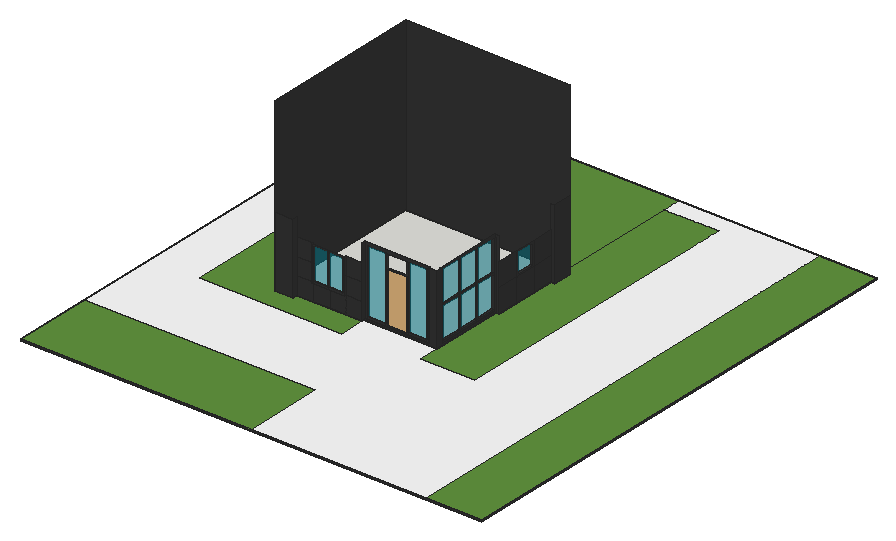
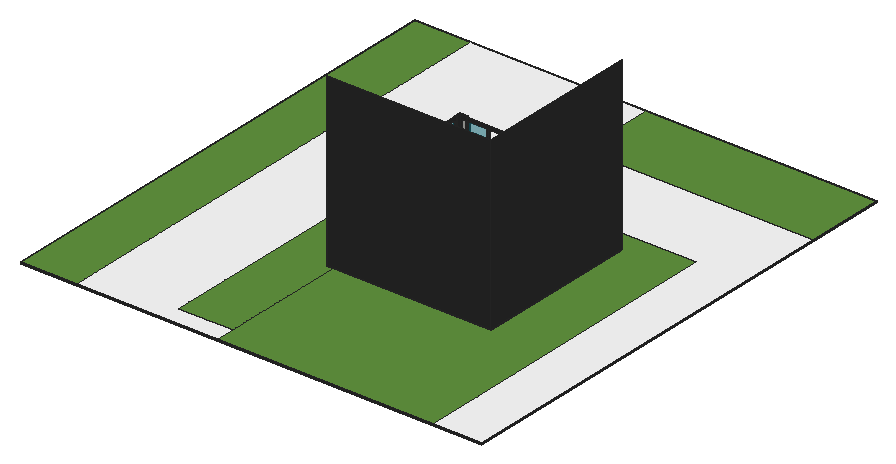
# SketchUp Ruby script. Lengths in inches.
U = 1.inch
M = Sketchup.active_model
def pt(a) = Geom::Point3d.new(a.map { |v| v * U })
def face(e, loops, mat)
  f = e.add_face(loops[0].map { |a| pt(a) })
  loops[1..].each { |l| e.add_face(l.map { |a| pt(a) }).erase! }
  f.material = f.back_material = mat if mat
  f
end
# faces: each face lists its corners as indices into pts; further lists are holes
def faces(e, pts, list, mat = nil) = list.each { |f| face(e, (f[0].is_a?(Array) ? f : [f]).map { |l| l.map { |i| pts[i] } }, mat) }
# xy, xz, yz: faces in a plane at the given z, y or x. An outline is a flat list of corners, or four numbers for a rectangle; further outlines are holes
def ring(l) = l.size == 4 ? [[l[0], l[1]], [l[2], l[1]], [l[2], l[3]], [l[0], l[3]]] : l.each_slice(2).to_a
def flat(e, list, mat, &to3) = list.each { |f| face(e, (f[0].is_a?(Array) ? f : [f]).map { |l| ring(l).map { |u, v| to3.(u, v) } }, mat) }
def xy(e, z, list, mat = nil) = flat(e, list, mat) { |x, y| [x, y, z] }
def xz(e, y, list, mat = nil) = flat(e, list, mat) { |x, z| [x, y, z] }
def yz(e, x, list, mat = nil) = flat(e, list, mat) { |y, z| [x, y, z] }
def lines(e, pts, list) = list.each { |a, b| e.add_line(pt(pts[a]), pt(pts[b])) }
# prism: a flat outline (further loops are holes) pulled along v
def prism(e, loops, v, mat = nil)
  f = face(e, loops, mat); d = Geom::Vector3d.new(v.map { |x| x * U })
  f.pushpull(f.normal.samedirection?(d) ? d.length : -d.length)
end
def box(e, o, s, mat = nil) = prism(e, [[o, [o[0] + s[0], o[1], o[2]], [o[0] + s[0], o[1] + s[1], o[2]], [o[0], o[1] + s[1], o[2]]]], [0, 0, s[2]], mat)
def at(x, y, z, deg = 0) = Geom::Transformation.translation(pt([x, y, z])) * Geom::Transformation.rotation(ORIGIN, Z_AXIS, deg.degrees)
def axes(o, x, y, z) = Geom::Transformation.new([*x, 0, *y, 0, *z, 0, *pt(o).to_a, 1])
def part(name) = M.definitions.add(name)
# library, detail: a bought-in or finely detailed component or shape, given as its bounding box
def library(name, o, s) = part(name).tap { |d| box(d.entities, o, s) }
def detail(e, o, s) = box(e.add_group.entities, o, s)
def put(e, d, t, mat = nil) = e.add_instance(d, t).tap { |i| i.material = mat if mat }
def group(e, t, mat = nil) = e.add_group.tap { |g| g.transformation = t; g.material = mat if mat }.entities
root = M.entities
M.materials.add("[0128_White]").color = [255, 255, 255]
M.materials.add("[0135_DarkGray]1").color = [53, 53, 53]
M.materials.add("[Grass Dark Green]").color = [97, 147, 63]
M.materials.add("[Translucent Glass Blue]1").color = [1, 149, 171]
M.materials["[Translucent Glass Blue]1"].alpha = 0.5
M.materials.add("[White Square Tile]").color = [255, 255, 255]
c1 = library("Glass door",[0,0,0],[43.79,7.72,89.79])
xy(root,-6,[[[0,0,1789.625,1912.5],[413.69,714.6875,485.69,714.6875,485.69,732.6875,738.69,732.6875,738.69,740.6875,1023.69,740.6875,1023.69,1026.6875,1035.69,1026.6875,1035.69,1278.6875,1049.69,1278.6875,1049.69,1350.6875,413.69,1350.6875]],[413.69,714.6875,413.69,1350.6875,1049.69,1350.6875,1049.69,1278.6875,1035.69,1278.6875,1035.69,1026.6875,1023.69,1026.6875,1023.69,740.6875,738.69,740.6875,738.69,732.6875,485.69,732.6875,485.69,714.6875]],"[0135_DarkGray]1")
xy(root,0,[[413.69,732.6875,738.69,732.6875,738.69,740.6875,1023.69,740.6875,1023.69,1350.6875,413.69,1350.6875]])
xy(root,0,[[413.69,714.6875,485.69,732.6875],[1023.69,1026.6875,1035.69,1026.6875,1035.69,1278.6875,1049.69,1278.6875,1049.69,1350.6875,1023.69,1350.6875]],"[0128_White]")
xy(root,0,[[0,0,894.8125,309.85],[1571.65,0,1789.625,1912.5],[[187.44,634.3125,738.69,634.3125,738.69,732.6875,485.69,732.6875,485.69,714.6875,413.69,714.6875,413.69,1350.6875,1023.69,1350.6875,1023.69,1912.5,187.44,1912.5],[413.69,714.6875,485.69,732.6875]],[1023.69,661.15,1235.57,661.15,1235.57,1840.4,1023.69,1840.4,1023.69,1350.6875,1049.69,1350.6875,1049.69,1278.6875,1035.69,1278.6875,1035.69,1026.6875,1023.69,1026.6875]],"[Grass Dark Green]")
xy(root,0,[[[894.8125,0,1571.65,0,1571.65,1912.5,1023.69,1912.5,1023.69,1840.4,1235.57,1840.4,1235.57,661.15,1023.69,661.15,1023.69,740.6875,738.69,740.6875,738.69,634.3125,187.44,634.3125,187.44,1912.5,0,1912.5,0,309.85,894.8125,309.85],[1023.69,1026.6875,1023.69,1350.6875,1049.69,1350.6875,1049.69,1278.6875,1035.69,1278.6875,1035.69,1026.6875]]],"[White Square Tile]")
xy(root,6,[[485.69,740.6875,738.69,745.6875]])
xy(root,6,[[738.69,740.6875,991.69,745.6875],[1018.69,762.6875,1023.69,1020.6875]],"[0135_DarkGray]1")
xy(root,12,[[750.69,745.6875,821.03,750.6875],[827.03,745.6875,903.36,750.6875],[909.36,745.6875,979.69,750.6875],[1013.69,774.6875,1018.69,856.6875],[1013.69,862.6875,1018.69,938.6875],
  [1013.69,944.6875,1018.69,1020.6875]],"[0135_DarkGray]1")
xy(root,67.89,[[548.94,728.6875,612.19,732.6875],[612.19,728.6875,675.44,732.6875]],"[0135_DarkGray]1")
xy(root,73.89,[[554.94,728.6875,609.19,732.6875],[615.19,728.6875,669.44,732.6875]],"[0135_DarkGray]1")
xy(root,96.52,[[1029.69,1116.6875,1035.69,1188.6875]],"[0135_DarkGray]1")
xy(root,132.78,[[1013.69,774.6875,1018.69,856.6875],[1013.69,862.6875,1018.69,938.6875],[1013.69,944.6875,1018.69,1020.6875]],"[0135_DarkGray]1")
xy(root,138.78,[[1013.69,774.6875,1018.69,856.6875],[1013.69,862.6875,1018.69,938.6875],[1013.69,944.6875,1018.69,1020.6875]],"[0135_DarkGray]1")
xy(root,175.04,[[1029.69,1116.6875,1035.69,1188.6875]],"[0135_DarkGray]1")
xz(root,0,[[0,-6,1789.625,0]],"[0135_DarkGray]1")
xz(root,714.6875,[[413.69,-6,485.69,0],[413.69,0,485.69,271.5625]],"[0135_DarkGray]1")
xz(root,728.6875,[[[548.94,67.89,675.44,203.67],[554.94,73.89,669.44,197.67]],[609.19,73.89,615.19,197.67]],"[0135_DarkGray]1")
xz(root,732.6875,[[485.69,-6,548.94,0],[548.94,-6,612.19,0],[612.19,-6,675.44,0],[675.44,-6,738.69,0],[485.69,0,548.94,67.89],
  [548.94,0,612.19,67.89],[612.19,0,675.44,67.89],[675.44,0,738.69,67.89],[485.69,67.89,548.94,135.78],[675.44,67.89,738.69,135.78],
  [485.69,135.78,548.94,203.67],[675.44,135.78,738.69,203.67]],"[0135_DarkGray]1")
xz(root,732.6875,[[554.94,73.89,609.19,197.67],[615.19,73.89,669.44,197.67]],"[Translucent Glass Blue]1")
xz(root,740.6875,[[738.69,-6,1023.69,0],[738.69,0,1023.69,0,1023.69,271.5625,991.69,271.5625,991.69,6,738.69,6]],"[0135_DarkGray]1")
xz(root,745.6875,[[[738.69,6,991.69,271.5625],[750.69,12,979.69,259.5625]],[821.03,12,827.03,12,827.03,204.96,903.36,204.96,903.36,12,909.36,12,909.36,259.5625,903.36,259.5625,903.36,211.2,827.03,211.2,827.03,259.5625,821.03,259.5625]],"[0135_DarkGray]1")
xz(root,750.6875,[[991.69,12,1001.69,259.5625]])
xz(root,750.6875,[[750.69,12,821.03,259.5625],[827.03,12,903.36,204.96],[909.36,12,979.69,259.5625]],"[Translucent Glass Blue]1")
xz(root,762.6875,[[1018.69,6,1023.69,271.5625]],"[0135_DarkGray]1")
xz(root,774.6875,[[1013.69,12,1018.69,132.78],[1013.69,138.78,1018.69,259.5625]],"[0135_DarkGray]1")
xz(root,856.6875,[[1013.69,12,1018.69,132.78],[1013.69,138.78,1018.69,259.5625]],"[0135_DarkGray]1")
xz(root,862.6875,[[1013.69,12,1018.69,132.78],[1013.69,138.78,1018.69,259.5625]],"[0135_DarkGray]1")
xz(root,938.6875,[[1013.69,12,1018.69,132.78],[1013.69,138.78,1018.69,259.5625]],"[0135_DarkGray]1")
xz(root,944.6875,[[1013.69,12,1018.69,132.78],[1013.69,138.78,1018.69,259.5625]],"[0135_DarkGray]1")
xz(root,1020.6875,[[1018.69,6,1023.69,6,1023.69,132.78,1013.69,132.78,1013.69,12,1018.69,12],[1018.69,132.78,1023.69,138.78],[1013.69,138.78,1023.69,259.5625]],"[0135_DarkGray]1")
xz(root,1026.6875,[[1023.69,-6,1035.69,0],[1023.69,0,1035.69,0,1035.69,271.5625,1018.69,271.5625,1018.69,259.5625,1023.69,259.5625]],"[0135_DarkGray]1")
xz(root,1116.6875,[[1029.69,96.52,1035.69,175.04]],"[0135_DarkGray]1")
xz(root,1188.6875,[[1029.69,96.52,1035.69,175.04]],"[0135_DarkGray]1")
xz(root,1278.6875,[[1035.69,-6,1049.69,0],[1035.69,0,1049.69,271.5625]],"[0135_DarkGray]1")
xz(root,1350.6875,[[413.69,-6,1049.69,0],[413.69,0,1049.69,660]],"[0135_DarkGray]1")
xz(root,1912.5,[[0,-6,1789.625,0]],"[0135_DarkGray]1")
yz(root,0,[[0,-6,1912.5,0]],"[0135_DarkGray]1")
yz(root,413.69,[[714.6875,-6,1350.6875,0],[714.6875,0,1350.6875,660]],"[0135_DarkGray]1")
yz(root,485.69,[[714.6875,-6,732.6875,0],[714.6875,0,732.6875,271.5625]],"[0135_DarkGray]1")
yz(root,548.94,[[728.6875,67.89,732.6875,135.78],[728.6875,135.78,732.6875,203.67]],"[0135_DarkGray]1")
yz(root,554.94,[[728.6875,73.89,732.6875,135.78],[728.6875,135.78,732.6875,197.67]],"[0135_DarkGray]1")
yz(root,609.19,[[728.6875,73.89,732.6875,197.67]],"[0135_DarkGray]1")
yz(root,615.19,[[728.6875,73.89,732.6875,197.67]],"[0135_DarkGray]1")
yz(root,669.44,[[728.6875,73.89,732.6875,135.78],[728.6875,135.78,732.6875,197.67]],"[0135_DarkGray]1")
yz(root,675.44,[[728.6875,67.89,732.6875,135.78],[728.6875,135.78,732.6875,203.67]],"[0135_DarkGray]1")
yz(root,738.69,[[732.6875,-6,740.6875,0],[732.6875,0,740.6875,0,740.6875,6,745.6875,6,745.6875,271.5625,732.6875,271.5625]],"[0135_DarkGray]1")
yz(root,750.69,[[745.6875,12,750.6875,259.5625]],"[0135_DarkGray]1")
yz(root,821.03,[[745.6875,12,750.6875,259.5625]],"[0135_DarkGray]1")
yz(root,827.03,[[745.6875,12,750.6875,204.96]],"[0135_DarkGray]1")
yz(root,903.36,[[745.6875,12,750.6875,204.96]],"[0135_DarkGray]1")
yz(root,909.36,[[745.6875,12,750.6875,259.5625]],"[0135_DarkGray]1")
yz(root,979.69,[[745.6875,12,750.6875,259.5625]],"[0135_DarkGray]1")
yz(root,991.69,[[745.6875,12,750.6875,259.5625]])
yz(root,991.69,[[740.6875,6,745.6875,271.5625]],"[0135_DarkGray]1")
yz(root,1013.69,[[774.6875,12,856.6875,132.78],[862.6875,12,938.6875,132.78],[944.6875,12,1020.6875,132.78],[774.6875,138.78,856.6875,259.5625],[862.6875,138.78,938.6875,259.5625],
  [944.6875,138.78,1020.6875,259.5625]],"[Translucent Glass Blue]1")
yz(root,1018.69,[[762.6875,6,1020.6875,6,1020.6875,12,774.6875,12,774.6875,259.5625,1026.6875,259.5625,1026.6875,271.5625,762.6875,271.5625],[856.6875,12,862.6875,259.5625],[938.6875,12,944.6875,259.5625],[774.6875,132.78,856.6875,138.78],[862.6875,132.78,938.6875,138.78],
  [944.6875,132.78,1020.6875,138.78]],"[0135_DarkGray]1")
yz(root,1023.69,[[740.6875,-6,1026.6875,0],[740.6875,0,1026.6875,0,1026.6875,259.5625,1020.6875,259.5625,1020.6875,6,762.6875,6,762.6875,271.5625,740.6875,271.5625]],"[0135_DarkGray]1")
yz(root,1029.69,[[1116.6875,96.52,1188.6875,175.04]],"[Translucent Glass Blue]1")
yz(root,1035.69,[[1026.6875,-6,1110.6875,0],[1110.6875,-6,1194.6875,0],[1194.6875,-6,1278.6875,0],[1026.6875,0,1110.6875,90.52],[1110.6875,0,1194.6875,90.52],
  [1194.6875,0,1278.6875,90.52],[1026.6875,90.52,1110.6875,181.04],[[1110.6875,90.52,1194.6875,181.04],[1116.6875,96.52,1188.6875,175.04]],[1194.6875,90.52,1278.6875,181.04]],"[0135_DarkGray]1")
yz(root,1049.69,[[1278.6875,-6,1350.6875,0],[1278.6875,0,1350.6875,271.5625]],"[0135_DarkGray]1")
yz(root,1789.625,[[0,-6,1912.5,0]],"[0135_DarkGray]1")
p = [[991.69,750.6875,0],[991.69,750.6875,12],[1013.69,762.6875,0],[1013.69,762.6875,271.5625],[485.69,745.6875,0],[485.69,745.6875,6],
  [991.69,745.6875,0],[991.69,745.6875,6],[1018.69,1020.6875,6],[1018.69,1026.6875,6],[1018.69,1026.6875,0]]
lines(root,p,[[0,1],[2,3],[4,5],[6,7],[8,9],[10,9]])
put(root,c1,axes([827.03,745.6875,12],[1.74328,0,0],[0,1,0],[0,0,2.14]))
